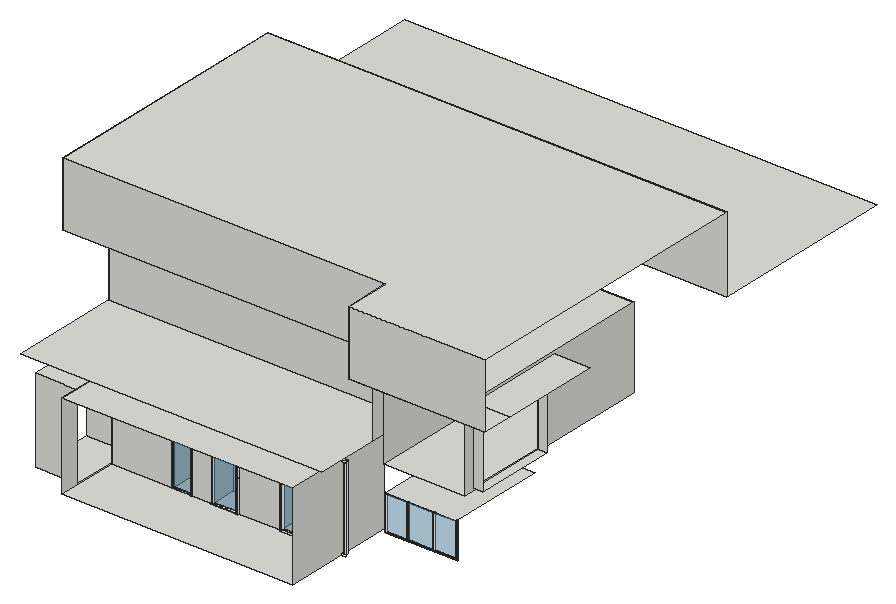
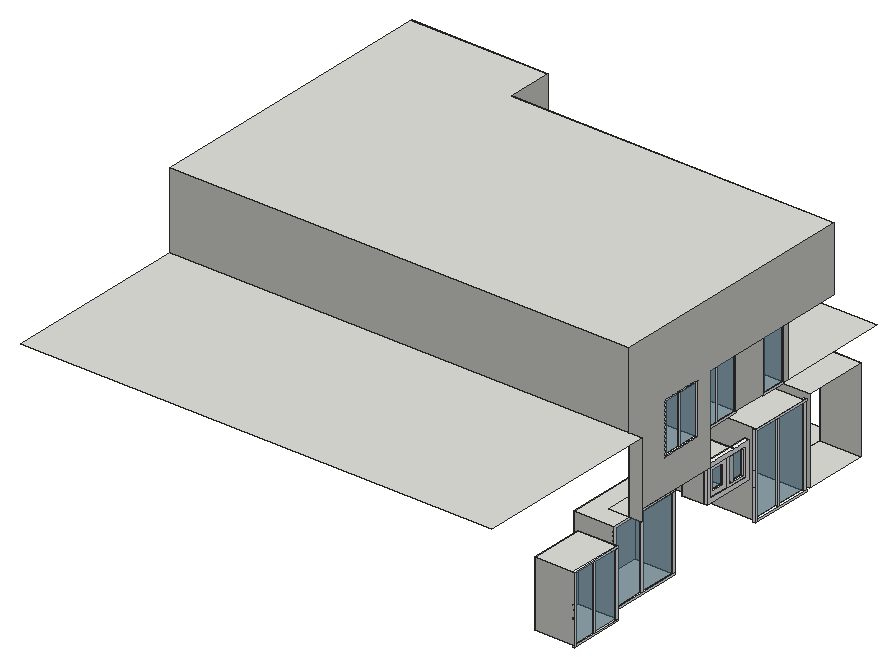
# SketchUp Ruby script. Lengths in inches.
U = 1.inch
M = Sketchup.active_model
def pt(a) = Geom::Point3d.new(a.map { |v| v * U })
def face(e, loops, mat)
  f = e.add_face(loops[0].map { |a| pt(a) })
  loops[1..].each { |l| e.add_face(l.map { |a| pt(a) }).erase! }
  f.material = f.back_material = mat if mat
  f
end
# faces: each face lists its corners as indices into pts; further lists are holes
def faces(e, pts, list, mat = nil) = list.each { |f| face(e, (f[0].is_a?(Array) ? f : [f]).map { |l| l.map { |i| pts[i] } }, mat) }
# xy, xz, yz: faces in a plane at the given z, y or x. An outline is a flat list of corners, or four numbers for a rectangle; further outlines are holes
def ring(l) = l.size == 4 ? [[l[0], l[1]], [l[2], l[1]], [l[2], l[3]], [l[0], l[3]]] : l.each_slice(2).to_a
def flat(e, list, mat, &to3) = list.each { |f| face(e, (f[0].is_a?(Array) ? f : [f]).map { |l| ring(l).map { |u, v| to3.(u, v) } }, mat) }
def xy(e, z, list, mat = nil) = flat(e, list, mat) { |x, y| [x, y, z] }
def xz(e, y, list, mat = nil) = flat(e, list, mat) { |x, z| [x, y, z] }
def yz(e, x, list, mat = nil) = flat(e, list, mat) { |y, z| [x, y, z] }
def lines(e, pts, list) = list.each { |a, b| e.add_line(pt(pts[a]), pt(pts[b])) }
# prism: a flat outline (further loops are holes) pulled along v
def prism(e, loops, v, mat = nil)
  f = face(e, loops, mat); d = Geom::Vector3d.new(v.map { |x| x * U })
  f.pushpull(f.normal.samedirection?(d) ? d.length : -d.length)
end
def box(e, o, s, mat = nil) = prism(e, [[o, [o[0] + s[0], o[1], o[2]], [o[0] + s[0], o[1] + s[1], o[2]], [o[0], o[1] + s[1], o[2]]]], [0, 0, s[2]], mat)
def at(x, y, z, deg = 0) = Geom::Transformation.translation(pt([x, y, z])) * Geom::Transformation.rotation(ORIGIN, Z_AXIS, deg.degrees)
def axes(o, x, y, z) = Geom::Transformation.new([*x, 0, *y, 0, *z, 0, *pt(o).to_a, 1])
def part(name) = M.definitions.add(name)
# library, detail: a bought-in or finely detailed component or shape, given as its bounding box
def library(name, o, s) = part(name).tap { |d| box(d.entities, o, s) }
def detail(e, o, s) = box(e.add_group.entities, o, s)
def put(e, d, t, mat = nil) = e.add_instance(d, t).tap { |i| i.material = mat if mat }
def group(e, t, mat = nil) = e.add_group.tap { |g| g.transformation = t; g.material = mat if mat }.entities
root = M.entities
M.materials.add("[Color_000]").color = [255, 255, 255]
M.materials.add("[Jade]").color = [77, 143, 110]
M.materials.add("[Translucent_Glass_Blue]1").color = [87, 149, 181]
M.materials["[Translucent_Glass_Blue]1"].alpha = 0.5
c1 = part("Group\#3")
xy(c1.entities,0,[[0,0,2.14,2.21]],"[Color_000]")
xy(c1.entities,1.67,[[2.14,0,29.96,2.21],[29.96,0,32.1,0.88],[32.1,0,64.19,2.21],[64.19,0,66.33,0.88]],"[Color_000]")
xy(c1.entities,84.95,[[2.14,0,29.96,2.21],[29.96,0,32.1,0.88],[32.1,0,64.19,2.21],[64.19,0,66.33,0.88]],"[Color_000]")
xy(c1.entities,86.61,[[0,0,66.33,2.21]],"[Color_000]")
xz(c1.entities,0,[[0,0,0,86.61,66.33,86.61,66.33,84.95,2.14,84.95,2.14,0],[2.14,0,66.33,1.67]],"[Color_000]")
xz(c1.entities,0.88,[[29.96,1.67,32.1,84.95],[64.19,1.67,66.33,84.95]],"[Color_000]")
xz(c1.entities,2.21,[[2.14,1.67,29.96,84.95],[32.1,1.67,64.19,84.95]],"[Translucent_Glass_Blue]1")
yz(c1.entities,0,[[0,0,2.21,32.8125],[0,32.8125,2.21,48.3],[0,48.3,2.21,86.61]],"[Color_000]")
yz(c1.entities,2.14,[[0,1.67,2.21,84.95]],"[Color_000]")
yz(c1.entities,29.96,[[0.88,1.67,2.21,84.95]],"[Color_000]")
yz(c1.entities,32.1,[[0.88,1.67,2.21,84.95]],"[Color_000]")
yz(c1.entities,64.19,[[0.88,1.67,2.21,84.95]],"[Color_000]")
yz(c1.entities,66.33,[[0.88,1.67,2.21,84.95]],"[Color_000]")
c2 = part("Group\#4")
xy(c2.entities,0,[[21.26,0,22.68,1.42]],"[Color_000]")
xy(c2.entities,1.42,[[0,0,1.42,0.57],[1.42,0,21.26,1.42]],"[Color_000]")
xy(c2.entities,72.28,[[0,0,1.42,0.57],[1.42,0,21.26,1.42]],"[Color_000]")
xy(c2.entities,73.7,[[0,0,21.26,1.42],[21.26,0,22.68,1.42]],"[Color_000]")
xz(c2.entities,0,[[0,0,21.26,1.42],[21.26,0,22.68,73.7],[0,72.28,21.26,73.7]],"[Color_000]")
xz(c2.entities,0.57,[[0,1.42,1.42,72.28]],"[Color_000]")
xz(c2.entities,1.42,[[21.26,0,22.68,73.7]],"[Color_000]")
xz(c2.entities,1.42,[[1.42,1.42,21.26,72.28]],"[Translucent_Glass_Blue]1")
yz(c2.entities,0,[[0.57,1.42,1.42,72.28]],"[Color_000]")
yz(c2.entities,1.42,[[0.57,1.42,1.42,72.28]],"[Color_000]")
yz(c2.entities,21.26,[[0,0,1.42,1.42],[0,1.42,1.42,72.28]],"[Color_000]")
yz(c2.entities,22.68,[[0,0,1.42,27.92],[0,27.92,1.42,41.1],[0,41.1,1.42,73.7]],"[Color_000]")
c3 = part("Group\#66")
xy(c3.entities,0,[[8858.27,0,9055.12,10236.22]],"[Color_000]")
xy(c3.entities,0,[[196.85,196.85,2755.91,10039.37],[2952.76,196.85,5905.51,10039.37],[6102.36,196.85,8858.27,10039.37]],"[Translucent_Glass_Blue]1")
xy(c3.entities,118.11,[[2755.91,196.85,2952.76,10039.37],[5905.51,196.85,6102.36,10039.37]],"[Color_000]")
xy(c3.entities,196.85,[[0,0,0,10236.22,8858.27,10236.22,8858.27,10039.37,196.85,10039.37,196.85,0],[196.85,0,8858.27,196.85],[8858.27,0,9055.12,10236.22]],"[Color_000]")
xz(c3.entities,0,[[0,0,196.85,196.85],[196.85,0,8858.27,196.85],[8858.27,0,9055.12,196.85]],"[Color_000]")
xz(c3.entities,196.85,[[196.85,0,2755.91,196.85],[2952.76,0,5905.51,196.85],[6102.36,0,8858.27,196.85],[2755.91,118.11,2952.76,196.85],[5905.51,118.11,6102.36,196.85]],"[Color_000]")
xz(c3.entities,10039.37,[[196.85,0,2755.91,196.85],[2952.76,0,5905.51,196.85],[6102.36,0,8858.27,196.85],[2755.91,118.11,2952.76,196.85],[5905.51,118.11,6102.36,196.85]],"[Color_000]")
xz(c3.entities,10236.22,[[0,0,8858.27,196.85],[8858.27,0,9055.12,196.85]],"[Color_000]")
yz(c3.entities,0,[[0,0,3877.95,196.85],[3877.95,0,5708.66,196.85],[5708.66,0,10236.22,196.85]],"[Color_000]")
yz(c3.entities,196.85,[[196.85,0,10039.37,196.85]],"[Color_000]")
yz(c3.entities,2755.91,[[196.85,0,10039.37,118.11]],"[Color_000]")
yz(c3.entities,2952.76,[[196.85,0,10039.37,118.11]],"[Color_000]")
yz(c3.entities,5905.51,[[196.85,0,10039.37,118.11]],"[Color_000]")
yz(c3.entities,6102.36,[[196.85,0,10039.37,118.11]],"[Color_000]")
yz(c3.entities,8858.27,[[0,0,196.85,196.85],[196.85,0,10039.37,196.85]],"[Color_000]")
yz(c3.entities,9055.12,[[0,0,3877.95,196.85],[3877.95,0,5708.66,196.85],[5708.66,0,10236.22,196.85]],"[Color_000]")
c4 = part("Group\#65")
xy(c4.entities,0,[[[275.59,275.59,3818.9,2244.09],[393.7,393.7,1909.45,2125.98],[2381.89,590.55,3503.9375,1929.13]]])
xy(c4.entities,0,[[[0,0,4094.49,2519.69],[275.59,275.59,3818.9,2244.09]]],"[Color_000]")
xy(c4.entities,0,[[393.7,393.7,1909.45,2125.98],[2381.89,590.55,3503.9375,1929.13]],"[Translucent_Glass_Blue]1")
xy(c4.entities,157.48,[[[2106.3,314.96,3779.53,2204.72],[2381.89,590.55,3503.9375,1929.13]]],"[Color_000]")
xy(c4.entities,196.85,[[[275.59,275.59,3818.9,2244.09],[2106.3,314.96,3779.53,2204.72],[393.7,393.7,1909.45,2125.98]]],"[Color_000]")
xy(c4.entities,236.22,[[[0,0,4094.49,2519.69],[275.59,275.59,3818.9,2244.09]]],"[Color_000]")
xz(c4.entities,0,[[0,0,4094.49,236.22]],"[Color_000]")
xz(c4.entities,275.59,[[275.59,0,3818.9,196.85],[275.59,196.85,3818.9,236.22]],"[Color_000]")
xz(c4.entities,314.96,[[2106.3,157.48,3779.53,196.85]],"[Color_000]")
xz(c4.entities,393.7,[[393.7,0,1909.45,196.85]],"[Color_000]")
xz(c4.entities,590.55,[[2381.89,0,3503.9375,157.48]],"[Color_000]")
xz(c4.entities,1929.13,[[2381.89,0,3503.9375,157.48]],"[Color_000]")
xz(c4.entities,2125.98,[[393.7,0,1909.45,196.85]],"[Color_000]")
xz(c4.entities,2204.72,[[2106.3,157.48,3779.53,196.85]],"[Color_000]")
xz(c4.entities,2244.09,[[275.59,0,3818.9,196.85],[275.59,196.85,3818.9,236.22]],"[Color_000]")
xz(c4.entities,2519.69,[[0,0,4094.49,236.22]],"[Color_000]")
yz(c4.entities,0,[[0,0,2519.69,236.22]],"[Color_000]")
yz(c4.entities,275.59,[[275.59,0,2244.09,196.85],[275.59,196.85,2244.09,236.22]],"[Color_000]")
yz(c4.entities,393.7,[[393.7,0,2125.98,196.85]],"[Color_000]")
yz(c4.entities,1909.45,[[393.7,0,2125.98,196.85]],"[Color_000]")
yz(c4.entities,2106.3,[[314.96,157.48,2204.72,196.85]],"[Color_000]")
yz(c4.entities,2381.89,[[590.55,0,1929.13,157.48]],"[Color_000]")
yz(c4.entities,3503.9375,[[590.55,0,1929.13,157.48]],"[Color_000]")
yz(c4.entities,3779.53,[[314.96,157.48,2204.72,196.85]],"[Color_000]")
yz(c4.entities,3818.9,[[275.59,0,2244.09,196.85],[275.59,196.85,2244.09,236.22]],"[Color_000]")
yz(c4.entities,4094.49,[[0,0,2519.69,236.22]],"[Color_000]")
xy(root,278.09,[[60,649.71,131.5,786.4]])
xy(root,281.62,[[134.85,198.52,547.79,198.52,547.79,402.08,437.9375,402.08,437.9375,308.89,357.55,308.89,357.55,354.21,316.01,354.21,316.01,308.89,279.63,308.89,279.63,354.21,244.58,354.21,244.58,308.89,134.85,308.89]])
xy(root,283.68,[[60,232.46,134.85,347.46]])
xy(root,284.7,[[60,360.8,242.875,469.11]])
xy(root,316.09,[[0,852.4375,71.4375,949.6875]])
xy(root,358.15,[[60,520.01,103.5625,578.58]])
xy(root,404.37,[[622.16,313.58,748.91,489.89]])
xy(root,414.78,[[60,649.71,131.5,786.4]])
xy(root,423.47,[[60,520.01,103.5625,578.58]])
xy(root,432.07,[[60,360.8,242.875,469.11]])
xy(root,433.4,[[0,852.4375,71.4375,949.6875]])
xy(root,434.87,[[60,232.46,134.85,347.46]])
xy(root,436.43,[[134.85,198.52,134.85,308.89,244.58,308.89,244.58,354.21,279.63,354.21,279.63,308.89,316.01,308.89,316.01,354.21,357.55,354.21,357.55,308.89,437.9375,308.89,437.9375,402.08,547.79,402.08,547.79,198.52]])
xy(root,448.41,[[22.75,618.52,60,798.52]])
xy(root,449.51,[[619.66,313.58,764.48,691.46]])
xy(root,453.66,[[764.48,331.61,782.0625,475.8]])
xy(root,480,[[60,198.52,600,397.08],[60,405.5,187.875,452.3125],[60,512.88,170.3125,591.88]])
xy(root,509.3,[[22.75,645.24,195.4375,719.24]])
xy(root,584.21,[[0,798.52,845.125,1134.21]])
xy(root,589.16,[[764.48,331.61,782.0625,475.8]])
xy(root,594.33,[[619.66,313.58,764.48,691.46]])
xy(root,594.5625,[[60,512.88,170.3125,591.88]])
xy(root,599.625,[[60,405.5,187.875,452.3125]])
xy(root,601.74,[[22.75,645.24,195.4375,719.24]])
xy(root,604.41,[[600,258.52,845.125,313.58],[22.75,339.83,60,618.52],[60,339.83,600,397.08]])
xy(root,720,[[600,258.52,845.125,258.52,845.125,798.52,22.75,798.52,22.75,339.83,600,339.83]])
xz(root,232.46,[[60,283.68,134.85,434.87]])
xz(root,258.52,[[600,604.41,845.125,720]])
xz(root,308.89,[[134.85,281.62,244.58,436.43],[279.63,281.62,316.01,436.43],[357.55,281.62,437.9375,436.43]])
xz(root,331.61,[[764.48,453.66,782.0625,589.16]])
xz(root,339.83,[[22.75,604.41,600,720]])
xz(root,347.46,[[60,283.68,134.85,434.87]])
xz(root,354.21,[[244.58,281.62,279.63,436.43],[316.01,281.62,357.55,436.43]])
xz(root,360.8,[[60,284.7,242.875,432.07]])
xz(root,397.08,[[60,480,600,604.41]])
xz(root,402.08,[[437.9375,281.62,547.79,436.43]])
xz(root,405.5,[[60,480,187.875,599.625]])
xz(root,452.3125,[[60,480,187.875,599.625]])
xz(root,469.11,[[60,284.7,242.875,432.07]])
xz(root,475.8,[[764.48,453.66,782.0625,589.16]])
xz(root,512.88,[[60,480,170.3125,594.5625]])
xz(root,520.01,[[60,358.15,103.5625,423.47]])
xz(root,578.58,[[60,358.15,103.5625,423.47]])
xz(root,591.88,[[60,480,170.3125,594.5625]])
xz(root,618.52,[[22.75,448.41,60,480],[22.75,480,60,604.41]])
xz(root,645.24,[[22.75,509.3,195.4375,601.74]])
xz(root,649.71,[[60,278.09,131.5,414.78]])
xz(root,691.46,[[619.66,449.51,764.48,594.33]])
xz(root,719.24,[[22.75,509.3,195.4375,601.74]])
xz(root,786.4,[[60,278.09,131.5,414.78]])
xz(root,798.52,[[0,448.41,22.75,584.21],[22.75,584.21,845.125,720]])
xz(root,852.4375,[[0,316.09,71.4375,433.4]])
xz(root,949.6875,[[0,316.09,71.4375,433.4]])
yz(root,22.75,[[[618.52,448.41,618.52,604.41,339.83,604.41,339.83,720,798.52,720,798.52,448.41],[645.24,509.3,719.24,601.74]]])
yz(root,60,[[397.08,480,397.08,604.41,618.52,604.41,618.52,480,591.88,480,591.88,594.5625,512.88,594.5625,512.88,480,452.3125,480,452.3125,599.625,405.5,599.625,405.5,480]])
yz(root,71.4375,[[852.4375,316.09,949.6875,433.4]])
yz(root,103.5625,[[520.01,358.15,578.58,423.47]])
yz(root,131.5,[[649.71,278.09,786.4,414.78]])
yz(root,134.85,[[198.52,281.62,308.89,281.62,308.89,283.68,232.46,283.68,232.46,434.87,308.89,434.87,308.89,436.43,198.52,436.43],[308.89,283.68,347.46,434.87]])
yz(root,170.3125,[[512.88,480,591.88,594.5625]])
yz(root,187.875,[[405.5,480,452.3125,599.625]])
yz(root,195.4375,[[645.24,509.3,719.24,601.74]])
yz(root,242.875,[[360.8,284.7,469.11,432.07]])
yz(root,244.58,[[308.89,281.62,354.21,436.43]])
yz(root,279.63,[[308.89,281.62,354.21,436.43]])
yz(root,316.01,[[308.89,281.62,354.21,436.43]])
yz(root,357.55,[[308.89,281.62,354.21,436.43]])
yz(root,437.9375,[[308.89,281.62,402.08,436.43]])
yz(root,547.79,[[198.52,281.62,402.08,436.43]])
yz(root,600,[[313.58,480,397.08,604.41],[258.52,604.41,339.83,720]])
yz(root,619.66,[[313.58,449.51,691.46,594.33]])
yz(root,764.48,[[[313.58,449.51,691.46,594.33],[331.61,453.66,475.8,589.16]]])
p = [[845.125,493.58,604.875],[845.125,313.58,604.41],[782.0625,313.58,604.41],[782.0625,493.58,604.875]]
faces(root,p,[[0,1,2,3]])
put(root,c1,axes([60,786.4,278.09],[0,-2.06072,0],[1,0,0],[0,0,1.57]))
put(root,c2,axes([314.59,307.32,280.2],[2.11,0,0],[0,2.11,0],[0,0,2.11]))
put(root,c2,axes([243.16,308.89,280.2],[1.60812,0,0],[0,1,0],[0,0,2.11]))
put(root,c1,axes([437.9375,307.17,281.62],[1.78,0,0],[0,1.78,0],[0,0,1.78]))
put(root,c1,axes([58.41,471.25,283.03],[0,-1.72,0],[1.72,0,0],[0,0,1.72]))
put(root,c1,axes([0,949.6875,313.48],[0,-1.46615,0],[1,0,0],[0,0,1.38462]))
put(root,c3,axes([620.74,315,341.11],[0.0144,0,0],[0,0,0.00618],[0,-0.0072,0]),"[Jade]")
put(root,c4,axes([65.51,486.67,423.51],[0,0.02245,0],[0,0,-0.02594],[-0.02917,0,0]),"[Jade]")
put(root,c1,axes([60,591.88,477.38],[0,-1.19101,0],[1,0,0],[0,0,1.38462]))
put(root,c2,axes([60,452.3125,478.58],[0,-2.0643,0],[1,0,0],[0,0,1.64]))
put(root,c1,axes([22.75,719.24,509.3],[0,-1.11563,0],[1,0,0],[0,0,1.06]))
